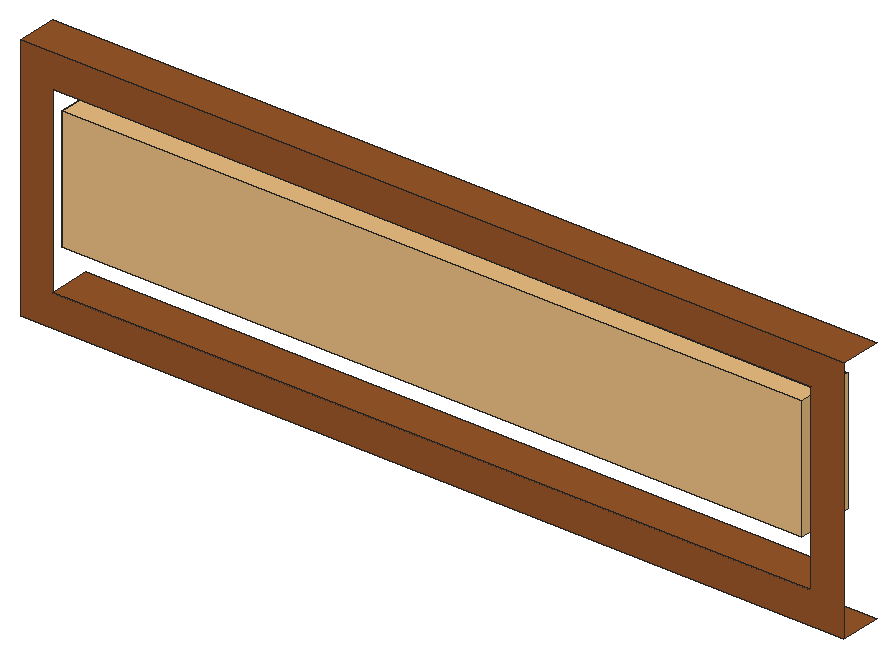
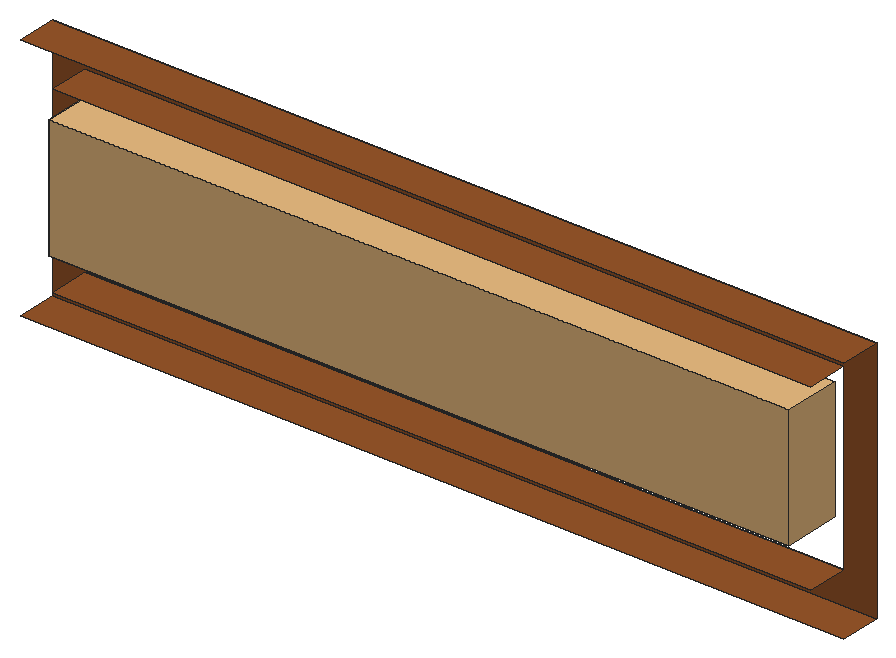
# SketchUp Ruby script. Lengths in inches.
U = 1.inch
M = Sketchup.active_model
def pt(a) = Geom::Point3d.new(a.map { |v| v * U })
def face(e, loops, mat)
  f = e.add_face(loops[0].map { |a| pt(a) })
  loops[1..].each { |l| e.add_face(l.map { |a| pt(a) }).erase! }
  f.material = f.back_material = mat if mat
  f
end
# faces: each face lists its corners as indices into pts; further lists are holes
def faces(e, pts, list, mat = nil) = list.each { |f| face(e, (f[0].is_a?(Array) ? f : [f]).map { |l| l.map { |i| pts[i] } }, mat) }
# xy, xz, yz: faces in a plane at the given z, y or x. An outline is a flat list of corners, or four numbers for a rectangle; further outlines are holes
def ring(l) = l.size == 4 ? [[l[0], l[1]], [l[2], l[1]], [l[2], l[3]], [l[0], l[3]]] : l.each_slice(2).to_a
def flat(e, list, mat, &to3) = list.each { |f| face(e, (f[0].is_a?(Array) ? f : [f]).map { |l| ring(l).map { |u, v| to3.(u, v) } }, mat) }
def xy(e, z, list, mat = nil) = flat(e, list, mat) { |x, y| [x, y, z] }
def xz(e, y, list, mat = nil) = flat(e, list, mat) { |x, z| [x, y, z] }
def yz(e, x, list, mat = nil) = flat(e, list, mat) { |y, z| [x, y, z] }
def lines(e, pts, list) = list.each { |a, b| e.add_line(pt(pts[a]), pt(pts[b])) }
# prism: a flat outline (further loops are holes) pulled along v
def prism(e, loops, v, mat = nil)
  f = face(e, loops, mat); d = Geom::Vector3d.new(v.map { |x| x * U })
  f.pushpull(f.normal.samedirection?(d) ? d.length : -d.length)
end
def box(e, o, s, mat = nil) = prism(e, [[o, [o[0] + s[0], o[1], o[2]], [o[0] + s[0], o[1] + s[1], o[2]], [o[0], o[1] + s[1], o[2]]]], [0, 0, s[2]], mat)
def at(x, y, z, deg = 0) = Geom::Transformation.translation(pt([x, y, z])) * Geom::Transformation.rotation(ORIGIN, Z_AXIS, deg.degrees)
def axes(o, x, y, z) = Geom::Transformation.new([*x, 0, *y, 0, *z, 0, *pt(o).to_a, 1])
def part(name) = M.definitions.add(name)
# library, detail: a bought-in or finely detailed component or shape, given as its bounding box
def library(name, o, s) = part(name).tap { |d| box(d.entities, o, s) }
def detail(e, o, s) = box(e.add_group.entities, o, s)
def put(e, d, t, mat = nil) = e.add_instance(d, t).tap { |i| i.material = mat if mat }
def group(e, t, mat = nil) = e.add_group.tap { |g| g.transformation = t; g.material = mat if mat }.entities
root = M.entities
M.materials.add("[Wood Cherry Original]1").color = [152, 86, 42]
c1 = library("KAVYA'S HOME",[2.54,0,0],[217.46,24.09,12])
xy(root,39.83,[[341.12,178.92,445.24,184.11]],"[Wood Cherry Original]1")
xy(root,43.94,[[345.23,178.92,441.13,184.11]],"[Wood Cherry Original]1")
xy(root,66.97,[[345.23,178.92,441.13,184.11]],"[Wood Cherry Original]1")
xy(root,71.08,[[341.12,178.92,445.24,184.11]],"[Wood Cherry Original]1")
xz(root,178.92,[[[341.12,39.83,445.24,71.08],[345.23,43.94,441.13,66.97]]],"[Wood Cherry Original]1")
put(root,c1,axes([345.23,178.92,49.48],[0.43051,0,0],[0,0,0.6391],[0,0.60953,0]))
